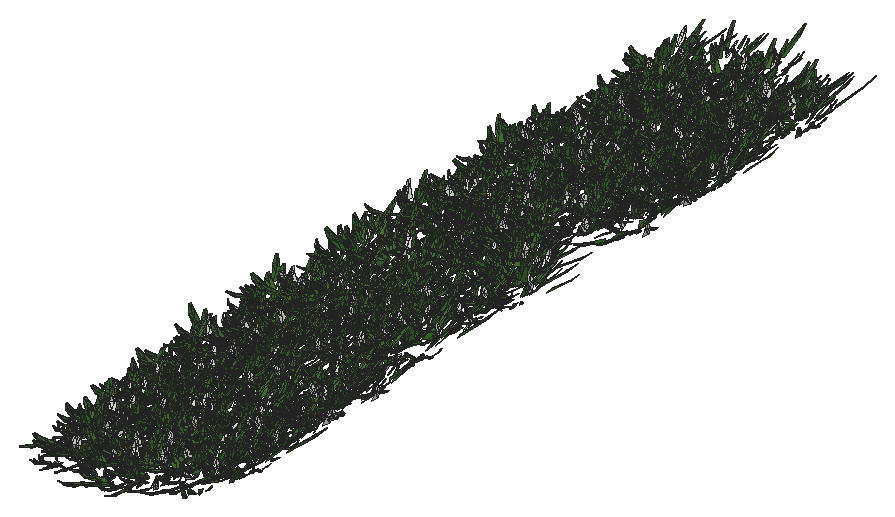
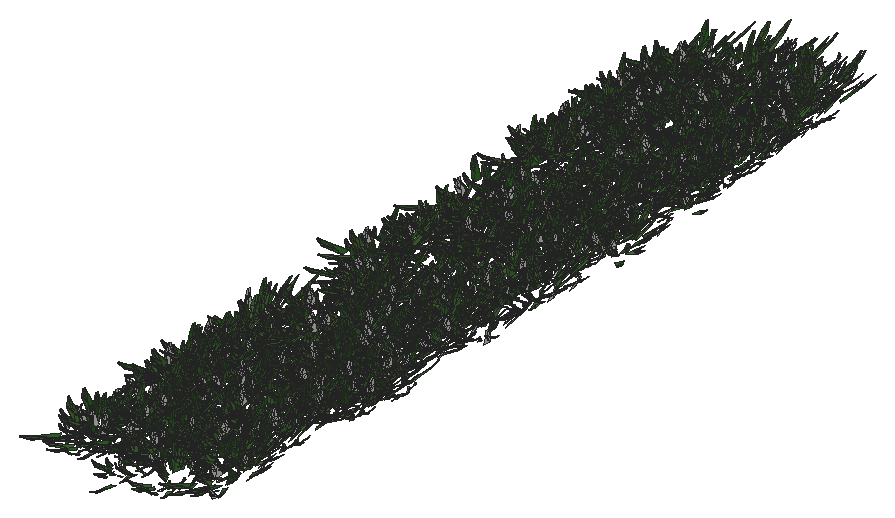
# SketchUp Ruby script. Lengths in inches.
U = 1.inch
M = Sketchup.active_model
def pt(a) = Geom::Point3d.new(a.map { |v| v * U })
def face(e, loops, mat)
  f = e.add_face(loops[0].map { |a| pt(a) })
  loops[1..].each { |l| e.add_face(l.map { |a| pt(a) }).erase! }
  f.material = f.back_material = mat if mat
  f
end
# faces: each face lists its corners as indices into pts; further lists are holes
def faces(e, pts, list, mat = nil) = list.each { |f| face(e, (f[0].is_a?(Array) ? f : [f]).map { |l| l.map { |i| pts[i] } }, mat) }
# xy, xz, yz: faces in a plane at the given z, y or x. An outline is a flat list of corners, or four numbers for a rectangle; further outlines are holes
def ring(l) = l.size == 4 ? [[l[0], l[1]], [l[2], l[1]], [l[2], l[3]], [l[0], l[3]]] : l.each_slice(2).to_a
def flat(e, list, mat, &to3) = list.each { |f| face(e, (f[0].is_a?(Array) ? f : [f]).map { |l| ring(l).map { |u, v| to3.(u, v) } }, mat) }
def xy(e, z, list, mat = nil) = flat(e, list, mat) { |x, y| [x, y, z] }
def xz(e, y, list, mat = nil) = flat(e, list, mat) { |x, z| [x, y, z] }
def yz(e, x, list, mat = nil) = flat(e, list, mat) { |y, z| [x, y, z] }
def lines(e, pts, list) = list.each { |a, b| e.add_line(pt(pts[a]), pt(pts[b])) }
# prism: a flat outline (further loops are holes) pulled along v
def prism(e, loops, v, mat = nil)
  f = face(e, loops, mat); d = Geom::Vector3d.new(v.map { |x| x * U })
  f.pushpull(f.normal.samedirection?(d) ? d.length : -d.length)
end
def box(e, o, s, mat = nil) = prism(e, [[o, [o[0] + s[0], o[1], o[2]], [o[0] + s[0], o[1] + s[1], o[2]], [o[0], o[1] + s[1], o[2]]]], [0, 0, s[2]], mat)
def at(x, y, z, deg = 0) = Geom::Transformation.translation(pt([x, y, z])) * Geom::Transformation.rotation(ORIGIN, Z_AXIS, deg.degrees)
def axes(o, x, y, z) = Geom::Transformation.new([*x, 0, *y, 0, *z, 0, *pt(o).to_a, 1])
def part(name) = M.definitions.add(name)
# library, detail: a bought-in or finely detailed component or shape, given as its bounding box
def library(name, o, s) = part(name).tap { |d| box(d.entities, o, s) }
def detail(e, o, s) = box(e.add_group.entities, o, s)
def put(e, d, t, mat = nil) = e.add_instance(d, t).tap { |i| i.material = mat if mat }
def group(e, t, mat = nil) = e.add_group.tap { |g| g.transformation = t; g.material = mat if mat }.entities
root = M.entities
M.materials.add("Material10").color = [48, 90, 38]
M.materials.add("Material11").color = [68, 110, 48]
M.materials.add("Material12").color = [48, 90, 48]
M.materials.add("Material13").color = [58, 110, 58]
M.materials.add("Material14").color = [58, 90, 38]
M.materials.add("Material15").color = [68, 100, 58]
M.materials.add("Material16").color = [48, 100, 38]
M.materials.add("Material9").color = [68, 110, 58]
c1 = part("grass00")
p = [[-0.6875,0.15,0],[-0.56,0.08,5.52],[-0.04,0.03,2.76],[0.48,-0.02,0],[0.35,-0.02,5.52],[-0.1,-0.14,5.52],
  [-0.12,0.65,8.37],[-0.42,0.65,8.37]]
faces(c1.entities,p,[[0,1,2,3],[3,2,4],[1,5,2],[5,4,2],[1,6,5],[4,5,6],[7,6,1]])
c2 = part("Group16\#1")
put(c2.entities,c1,axes([1.44,-0.61,-0.01],[0.05352,0.12609,0],[-0.10704,0.04543,0.07239],[0.06664,-0.02828,0.11628]),"Material12")
put(c2.entities,c1,axes([0.76,-0.15,-0.01],[0.04676,0.24062,0],[-0.23162,0.04501,0.06642],[0.0652,-0.01267,0.23595]),"Material9")
put(c2.entities,c1,axes([0.79,0.01,-0.01],[-0.00606,0.34651,0],[-0.34381,-0.00602,0.0432],[0.04319,0.00076,0.34386]))
put(c2.entities,c1,axes([1,0.23,-0.01],[-0.07192,0.31144,0],[-0.28722,-0.06632,0.1236],[0.12043,0.02781,0.29478]),"Material11")
put(c2.entities,c1,axes([1.66,0.77,-0.01],[-0.13828,0.29651,0],[-0.21551,-0.1005,0.22471],[0.20365,0.09498,0.23779]),"Material16")
put(c2.entities,c1,axes([0.6875,0.52,-0.01],[-0.18126,0.24051,0],[-0.22746,-0.17142,0.09788],[0.07817,0.05891,0.28481]),"Material11")
put(c2.entities,c1,axes([0.68,0.78,-0.01],[-0.215,0.18688,0],[-0.12385,-0.14248,0.21334],[0.13995,0.16101,0.18878]),"Material9")
put(c2.entities,c1,axes([0.56,1,-0.01],[-0.13756,0.07624,0],[-0.06159,-0.11112,0.0927],[0.04494,0.08108,0.12705]),"Material11")
put(c2.entities,c1,axes([0.2,0.64,-0.01],[-0.23729,0.07254,0],[-0.05711,-0.18681,0.153],[0.04473,0.14632,0.19535]),"Material16")
put(c2.entities,c1,axes([0.0625,0.72,-0.01],[-0.28874,0.02525,0],[-0.02179,-0.24916,0.14647],[0.01276,0.14591,0.25012]),"Material9")
put(c2.entities,c1,axes([-0.08,0.62,-0.01],[-0.34089,-0.04187,0],[0.03255,-0.26504,0.216],[-0.02633,0.21439,0.26703]),"Material16")
put(c2.entities,c1,axes([-0.34,0.98,-0.01],[-0.14314,-0.0493,0],[0.04397,-0.12769,0.06843],[-0.02228,0.0647,0.13505]),"Material16")
put(c2.entities,c1,axes([-0.87,1.45,-0.01],[-0.23488,-0.14114,0],[0.13761,-0.22901,0.06087],[-0.03135,0.05217,0.26717]))
put(c2.entities,c1,axes([-0.72,0.77,-0.01],[-0.14208,-0.13251,0],[0.07209,-0.0773,0.16301],[-0.11118,0.11922,0.1057]),"Material16")
put(c2.entities,c1,axes([-0.62,0.43,-0.01],[-0.14845,-0.21203,0],[0.18654,-0.13061,0.12304],[-0.10079,0.07057,0.22772]),"Material9")
put(c2.entities,c1,axes([-0.68,0.29,-0.01],[-0.13639,-0.32136,0],[0.31723,-0.13464,0.05579],[-0.05136,0.0218,0.34462]),"Material10")
put(c2.entities,c1,axes([-0.64,0.125,-0.01],[-0.0458,-0.23569,0],[0.22124,-0.043,0.08276],[-0.08124,0.01579,0.22538]),"Material13")
put(c2.entities,c1,axes([-1.6,-0.03,-0.01],[0.00576,-0.32897,0],[0.27526,0.00482,0.18018],[-0.18015,-0.00315,0.2753]),"Material11")
put(c2.entities,c1,axes([-1.36,-0.31,-0.01],[0.05718,-0.24765,0],[0.18172,0.04196,0.17267],[-0.16825,-0.03885,0.1865]),"Material16")
put(c2.entities,c1,axes([-1.54,-0.72,-0.01],[0.06537,-0.14017,0],[0.13555,0.06321,0.03939],[-0.0357,-0.01665,0.14956]))
put(c2.entities,c1,axes([-1.19,-0.9,-0.01],[0.09597,-0.12735,0],[0.11214,0.08451,0.07557],[-0.06035,-0.04548,0.14042]),"Material15")
put(c2.entities,c1,axes([-0.47,-0.54,-0.01],[0.11588,-0.10072,0],[0.0618,0.0711,0.12124],[-0.07953,-0.0915,0.0942]))
put(c2.entities,c1,axes([-0.47,-0.84,-0.01],[0.11927,-0.0661,0],[0.06603,0.11913,0.00646],[-0.00313,-0.00565,0.13621]),"Material11")
put(c2.entities,c1,axes([-0.38,-1.24,-0.01],[0.28037,-0.08571,0],[0.0618,0.20215,0.20315],[-0.05939,-0.19428,0.21139]),"Material15")
put(c2.entities,c1,axes([-0.06,-0.66,-0.01],[0.22719,-0.01987,0],[0.01247,0.14255,0.17758],[-0.01547,-0.17691,0.1431]),"Material14")
put(c2.entities,c1,axes([0.11,-0.89,-0.01],[0.14882,0.01828,0],[-0.01058,0.08611,0.12229],[0.01491,-0.12138,0.08676]),"Material12")
put(c2.entities,c1,axes([0.25,-0.72,-0.01],[0.20481,0.07053,0],[-0.06206,0.18022,0.10291],[0.03351,-0.0973,0.1906]),"Material12")
put(c2.entities,c1,axes([0.85,-1.42,-0.01],[0.16481,0.09904,0],[-0.09472,0.15762,0.05616],[0.02893,-0.04814,0.18389]),"Material11")
put(c2.entities,c1,axes([1.01,-1.09,-0.01],[0.21858,0.20385,0],[-0.17495,0.1876,0.15339],[0.10462,-0.11218,0.25652]),"Material16")
put(c2.entities,c1,axes([1.01,-0.71,-0.01],[0.08733,0.12473,0],[-0.06445,0.04512,0.13037],[0.1068,-0.07477,0.07867]),"Material12")
c3 = part("Group15\#1")
put(c3.entities,c2,at(0,0,0))
c4 = part("3darcstudiotree_grass00\#1")
put(c4.entities,c3,at(0,0,0))
put(root,c4,axes([911.62,507.39,12.99],[0.34,5.72697,0],[-2.64342,0.82003,-0.02967],[-0.12642,0.03922,1.57371]))
put(root,c4,axes([901.09,511.3,12.99],[1.82287,-4.38693,0],[2.28516,4.96154,-0.03691],[0.11809,0.2564,1.90749]))
put(root,c4,axes([899.3,512.19,12.99],[2.37795,-5.62127,0],[2.1378,4.72541,-0.03201],[0.10645,0.23529,1.88682]))
put(root,c4,axes([919.3,511.88,12.99],[2.50076,5.4884,0],[-2.31392,5.50908,-0.04664],[-0.12544,0.29866,1.77978]))
put(root,c4,axes([922.17,511.91,12.99],[-1.24752,4.90683,0],[-3.03213,-4.02809,-0.02835],[-0.08818,-0.11714,1.73088]))
put(root,c4,axes([905.31,513.99,12.99],[-2.27824,4.59704,0],[-2.30362,-5.96536,-0.01862],[-0.04923,-0.12749,1.90809]))
put(root,c4,axes([914.17,516,12.99],[-2.60594,2.85858,0],[-1.16429,-5.546,-0.02803],[-0.06327,-0.30136,1.92571]))
put(root,c4,axes([930.93,518.19,12.99],[3.35601,0.53822,0],[-0.22532,7.34135,-0.05051],[-0.0153,0.49834,1.91076]))
put(root,c4,axes([895.08,521.84,12.99],[-1.92991,-4.90294,0],[2.14831,-4.41857,-0.02928],[0.07464,-0.15352,1.35967]))
put(root,c4,axes([905.65,523.44,12.99],[-2.63848,-1.86566,0],[1.00702,-7.44154,-0.06046],[0.05687,-0.42027,1.48798]))
put(root,c4,axes([926,523.89,12.99],[-3.10548,-1.18132,0],[0.44818,-6.15625,-0.03971],[0.0257,-0.35297,1.4765]))
put(root,c4,axes([897.49,523.26,12.99],[-1.16449,5.45396,0],[-2.90449,-3.2404,-0.02753],[-0.10274,-0.11462,1.84121]))
put(root,c4,axes([914.51,526.17,12.99],[2.93419,-3.82384,0],[1.37593,5.51683,-0.05304],[0.12846,0.51506,1.86337]))
put(root,c4,axes([934.71,526.73,12.99],[2.24209,2.16707,0],[-1.0186,5.50663,-0.04149],[-0.08583,0.46398,1.90578]))
put(root,c4,axes([931.51,530.82,12.99],[-0.7426,-6.639,0],[2.915,-1.7037,-0.04783],[0.18057,-0.10554,1.6084]))
put(root,c4,axes([934.66,531.55,12.99],[2.98703,2.46119,0],[-1.07432,6.81293,-0.05978],[-0.06973,0.44222,1.49495]))
put(root,c4,axes([914.19,532.2,12.99],[3.29113,-0.43396,0],[0.16052,6.36086,-0.03809],[0.0103,0.40827,1.79573]))
put(root,c4,axes([926.06,532.53,12.99],[2.54195,2.07367,0],[-1.08806,6.96921,-0.03925],[-0.03862,0.24738,1.29995]))
put(root,c4,axes([917.6,531.75,12.99],[0.49074,6.09032,0],[-2.95531,1.24429,-0.0472],[-0.16503,0.06948,1.46547]))
put(root,c4,axes([897.78,535.97,12.99],[1.52125,-4.69601,0],[2.1276,3.60136,-0.04843],[0.18496,0.31307,1.72564]))
put(root,c4,axes([903.64,536.54,12.99],[2.39249,-2.44782,0],[1.16829,5.96659,-0.04939],[0.0929,0.47446,1.80606]))
put(root,c4,axes([895.21,535.38,12.99],[-0.41215,7.13038,0],[-3.37299,-1.01874,-0.03274],[-0.10036,-0.03031,1.44297]))
put(root,c4,axes([911.05,535.47,12.99],[-1.79373,6.75105,0],[-2.77607,-3.8541,-0.06137],[-0.17197,-0.23875,1.46064]))
put(root,c4,axes([923.03,540.81,12.99],[2.70825,1.08108,0],[-0.55903,7.3176,-0.04039],[-0.02179,0.2852,1.39779]))
put(root,c4,axes([926.1,541.03,12.99],[3.0266,-0.27277,0],[0.11405,6.61218,-0.03451],[0.00641,0.37148,1.8714]))
put(root,c4,axes([896.8,540.54,12.99],[0.57317,6.39839,0],[-3.07282,1.43831,-0.02758],[-0.10194,0.04772,1.62317]))
put(root,c4,axes([894.13,542.98,12.99],[-0.04355,-5.68696,0],[3.06634,-0.12269,-0.04239],[0.1434,-0.00574,1.42343]))
put(root,c4,axes([935.43,543.85,12.99],[1.14678,-5.5994,0],[2.21293,2.36815,-0.04141],[0.22096,0.23646,1.97468]))
put(root,c4,axes([910.25,543.03,12.99],[-0.07356,6.6061,0],[-2.87925,-0.16752,-0.03168],[-0.13306,-0.00774,1.66016]))
put(root,c4,axes([916.99,545.44,12.99],[-0.22644,-5.7932,0],[3.1204,-0.63732,-0.01785],[0.07882,-0.0161,1.90542]))
put(root,c4,axes([901.99,546.02,12.99],[-2.22727,-5.99191,0],[2.4648,-4.78734,-0.06095],[0.18437,-0.35809,1.76096]))
put(root,c4,axes([908.8,549.42,12.99],[-1.36063,-6.84812,0],[2.89693,-3.00754,-0.02239],[0.08865,-0.09204,1.89813]))
put(root,c4,axes([922.76,551.22,12.99],[2.82961,-3.8496,0],[1.56723,6.01934,-0.02674],[0.04894,0.18795,1.50406]))
put(root,c4,axes([925.56,552.73,12.99],[2.24091,-5.60604,0],[1.99594,4.16889,-0.04297],[0.12661,0.26444,1.48019]))
put(root,c4,axes([893.13,553.17,12.99],[1.46268,-6.84801,0],[2.66295,2.97202,-0.03421],[0.14319,0.15981,1.89316]))
put(root,c4,axes([933.37,554.94,12.99],[-1.60421,-6.26587,0],[2.10282,-2.81311,-0.0221],[0.10402,-0.13915,1.82262]))
put(root,c4,axes([899.48,555.6,12.99],[-0.27492,-6.2516,0],[2.80374,-0.64426,-0.02999],[0.1475,-0.03389,1.91089]))
put(root,c4,axes([901.93,554.68,12.99],[-2.10162,2.80691,0],[-1.6179,-6.32971,-0.05376],[-0.08517,-0.33321,1.38154]))
put(root,c4,axes([931.97,558.13,12.99],[1.20273,-5.08222,0],[2.87348,3.55326,-0.03985],[0.11745,0.14524,1.5017]))
put(root,c4,axes([910.82,559.6,12.99],[2.65553,-1.98837,0],[0.86174,6.01359,-0.03684],[0.04886,0.34099,1.61813]))
put(root,c4,axes([919.3,559.79,12.99],[-0.92876,-5.81291,0],[2.33925,-1.95294,-0.03784],[0.17266,-0.14414,1.65933]))
put(root,c4,axes([899.22,560.83,12.99],[0.14872,-5.87734,0],[2.84203,0.37577,-0.03098],[0.1244,0.01645,1.57088]))
put(root,c4,axes([893.03,560.92,12.99],[-0.76721,-6.56598,0],[2.80308,-1.71142,-0.04991],[0.16056,-0.09803,1.32514]))
put(root,c4,axes([901.87,563.86,12.99],[0.86779,-6.44688,0],[3.29606,2.31828,-0.02541],[0.07611,0.05354,1.48254]))
put(root,c4,axes([925.49,564.01,12.99],[3.00912,-1.86696,0],[0.83394,7.02336,-0.0215],[0.02203,0.18551,1.70776]))
put(root,c4,axes([933.42,564.83,12.99],[-2.81152,-3.41489,0],[1.39335,-5.99415,-0.03648],[0.07534,-0.32411,1.79293]))
put(root,c4,axes([913.24,567.95,12.99],[2.91119,-3.41984,0],[1.58451,7.04797,-0.04443],[0.05964,0.26528,1.39643]))
put(root,c4,axes([930.81,568.44,12.99],[1.07755,-6.0652,0],[2.75492,2.55744,-0.04502],[0.19028,0.17664,1.86083]))
put(root,c4,axes([898.57,570.125,12.99],[0.66031,-7.75823,0],[2.98052,1.3255,-0.02432],[0.08896,0.03956,1.55217]))
put(root,c4,axes([903.51,568.01,12.99],[-2.55136,-0.37019,0],[0.21266,-7.65835,-0.04372],[0.00789,-0.28423,1.31241]))
put(root,c4,axes([892.51,568.625,12.99],[-2.70337,4.4882,0],[-1.55371,-4.89002,-0.02785],[-0.08332,-0.26224,1.84622]))
put(root,c4,axes([906.42,572.39,12.99],[0.82047,6.51109,0],[-2.65358,1.74721,-0.02733],[-0.11397,0.07504,1.64375]))
put(root,c4,axes([934.53,573.93,12.99],[-1.61582,-5.04917,0],[2.30469,-3.85382,-0.02018],[0.07529,-0.12589,1.81061]))
put(root,c4,axes([909.06,573.86,12.99],[1.03892,6.48849,0],[-2.96707,2.4824,-0.03042],[-0.10595,0.08864,1.60735]))
put(root,c4,axes([917.76,577.75,12.99],[2.83159,1.20572,0],[-0.46618,5.72066,-0.03922],[-0.03004,0.36868,1.46066]))
put(root,c4,axes([927.84,578.64,12.99],[-0.05016,-6.74869,0],[3.47924,-0.13511,-0.0635],[0.25664,-0.00997,1.92948]))
put(root,c4,axes([903.48,577.58,12.99],[-2.8288,-1.01098,0],[0.5257,-7.68597,-0.04342],[0.02399,-0.35073,1.66984]))
put(root,c4,axes([907.71,577.89,12.99],[0.7383,7.4918,0],[-2.86561,1.4756,-0.04632],[-0.17959,0.09248,1.6013]))
put(root,c4,axes([898.29,578.13,12.99],[-3.47147,0.94023,0],[-0.34005,-6.56028,-0.03012],[-0.01166,-0.22504,1.30483]))
put(root,c4,axes([913.85,580.83,12.99],[2.85458,-2.4144,0],[0.90082,5.56514,-0.04569],[0.07926,0.48966,1.78027]))
put(root,c4,axes([895.07,582.8,12.99],[-0.07151,5.57846,0],[-2.5198,-0.16879,-0.04664],[-0.191,-0.01279,1.41669]))
put(root,c4,axes([902.39,589.33,12.99],[-2.87948,-2.17383,0],[0.90398,-6.25682,-0.04962],[0.07103,-0.49164,1.8049]))
put(root,c4,axes([919.75,591.55,12.99],[2.81213,-4.07835,0],[1.6403,5.90987,-0.04672],[0.11008,0.39661,1.84728]))
put(root,c4,axes([913.87,591,12.99],[-1.55553,-5.63634,0],[2.69451,-3.88567,-0.04882],[0.13072,-0.18851,1.38366]))
put(root,c4,axes([926.78,593.01,12.99],[0.94413,-7.19204,0],[2.66579,1.82856,-0.0465],[0.16992,0.11655,1.45674]))
put(root,c4,axes([923.21,591.68,12.99],[2.50014,4.15141,0],[-1.81588,5.71425,-0.05492],[-0.12483,0.39281,1.63919]))
put(root,c4,axes([890.46,595.94,12.99],[-1.39258,5.37899,0],[-2.78969,-3.77383,-0.04665],[-0.1335,-0.18059,1.47851]))
put(root,c4,axes([931.64,597.86,12.99],[3.08666,3.01957,0],[-1.37734,7.35682,-0.06274],[-0.09879,0.52768,1.92197]))
put(root,c4,axes([922.87,601.0625,12.99],[3.40345,0.80319,0],[-0.35208,7.79564,-0.06196],[-0.02083,0.46114,1.53928]))
put(root,c4,axes([896.75,599.38,12.99],[-2.37919,1.70232,0],[-0.98908,-7.22313,-0.0251],[-0.02634,-0.19235,1.59541]))
put(root,c4,axes([910.33,600.22,12.99],[1.27071,7.43264,0],[-2.73445,2.44274,-0.05423],[-0.17184,0.15351,1.37014]))
put(root,c4,axes([914.18,601.01,12.99],[-2.71794,-2.84239,0],[1.0724,-5.35819,-0.02741],[0.0602,-0.30081,1.86713]))
put(root,c4,axes([907.29,602.4375,12.99],[3.09734,3.11798,0],[-1.07985,5.60512,-0.04159],[-0.06485,0.33661,1.42181]))
put(root,c4,axes([901.5625,600.88,12.99],[-0.67912,7.33073,0],[-3.23912,-1.56795,-0.05285],[-0.196,-0.09488,1.72177]))
put(root,c4,axes([895.03,602.25,12.99],[2.06342,5.41056,0],[-1.85953,3.70556,-0.0286],[-0.1154,0.22996,1.81122]))
put(root,c4,axes([921.49,605.92,12.99],[1.54134,-4.78126,0],[2.32684,3.91946,-0.04551],[0.15187,0.25581,1.64335]))
put(root,c4,axes([914.17,605.18,12.99],[-1.50632,-4.69201,0],[2.73865,-4.59409,-0.05528],[0.17049,-0.28599,1.78248]))
put(root,c4,axes([919.71,607.39,12.99],[-3.46773,-1.02932,0],[0.4256,-7.49196,-0.02421],[0.01142,-0.20095,1.66024]))
put(root,c4,axes([910.52,608.8,12.99],[-2.49845,-5.44109,0],[2.40238,-5.76411,-0.03405],[0.07195,-0.17263,1.46358]))
put(root,c4,axes([894.73,610.01,12.99],[-0.0959,-6.54768,0],[3.1318,-0.23968,-0.02714],[0.09123,-0.00698,1.44559]))
put(root,c4,axes([901.81,609.875,12.99],[-2.1387,-4.22142,0],[1.73135,-4.58332,-0.01919],[0.06882,-0.18218,1.99409]))
put(root,c4,axes([929.98,611.28,12.99],[-0.93481,-5.37778,0],[2.82075,-2.56208,-0.04918],[0.14755,-0.13402,1.34418]))
put(root,c4,axes([917.01,616.94,12.99],[2.59771,-2.31669,0],[0.88695,5.19669,-0.03886],[0.06413,0.37576,1.52001]))
put(root,c4,axes([923.46,615.26,12.99],[-2.73622,0.78622,0],[-0.41112,-7.47622,-0.04842],[-0.02602,-0.47315,1.94818]))
put(root,c4,axes([930.31,619.48,12.99],[0.40616,-5.59706,0],[3.26818,1.23923,-0.06063],[0.20259,0.07682,1.53907]))
put(root,c4,axes([899.28,625.21,12.99],[1.48607,-6.00699,0],[2.71444,3.50888,-0.04614],[0.13946,0.18028,1.48544]))
put(root,c4,axes([928.17,625.99,12.99],[2.65845,-2.85345,0],[1.05816,5.15125,-0.03796],[0.07227,0.35184,1.52986]))
put(root,c4,axes([891.27,623.87,12.99],[0.1348,6.56883,0],[-3.04635,0.32665,-0.04808],[-0.19581,0.021,1.70557]))
put(root,c4,axes([911.5625,625.78,12.99],[1.96904,6.36442,0],[-2.63699,4.26294,-0.03132],[-0.10336,0.16709,1.7905]))
put(root,c4,axes([902.68,625.72,12.99],[-1.44847,7.20412,0],[-2.84419,-2.98807,-0.02861],[-0.11414,-0.11991,1.88512]))
put(root,c4,axes([917.68,628.26,12.99],[1.92859,6.40127,0],[-2.1329,3.35776,-0.04649],[-0.14033,0.22092,1.30192]))
put(root,c4,axes([892.55,628.5,12.99],[0.7965,6.40774,0],[-3.08556,2.00411,-0.01918],[-0.07901,0.05132,1.88463]))
put(root,c4,axes([933.56,634.16,12.99],[3.0297,-0.61474,0],[0.27475,7.07526,-0.01913],[0.00739,0.1902,1.86132]))
put(root,c4,axes([909.38,635.46,12.99],[2.96081,2.71039,0],[-1.11902,6.38738,-0.05201],[-0.08237,0.47016,1.75905]))
put(root,c4,axes([899.58,638.61,12.99],[-2.68453,-4.05111,0],[1.51474,-5.2449,-0.0411],[0.0862,-0.29848,1.43569]))
put(root,c4,axes([927.57,637.76,12.99],[-0.5928,7.42861,0],[-3.44276,-1.43553,-0.02378],[-0.09545,-0.0398,1.95907]))
put(root,c4,axes([899.32,642.41,12.99],[2.59926,-1.54725,0],[0.69692,6.11752,-0.03218],[0.02822,0.24776,1.32043]))
put(root,c4,axes([927.82,642.72,12.99],[3.30378,0.12998,0],[-0.05244,6.96435,-0.04862],[-0.00279,0.3699,1.39123]))
put(root,c4,axes([911.83,642.75,12.99],[-1.81939,4.62689,0],[-2.16643,-4.4513,-0.05045],[-0.13948,-0.28658,1.48531]))
put(root,c4,axes([918.25,646.97,12.99],[1.07125,-5.88046,0],[2.56502,2.44161,-0.04485],[0.17282,0.1645,1.59096]))
put(root,c4,axes([923.6875,649.01,12.99],[2.65984,-5.15497,0],[1.88895,5.09277,-0.04452],[0.14052,0.37886,1.95574]))
put(root,c4,axes([913.17,646.6875,12.99],[0.28785,6.1866,0],[-3.00356,0.73023,-0.05804],[-0.19462,0.04732,1.39706]))
put(root,c4,axes([903.36,648.48,12.99],[-0.63085,-5.64288,0],[2.60325,-1.52071,-0.03508],[0.17624,-0.10295,1.91126]))
put(root,c4,axes([890.6,648.84,12.99],[1.84408,4.39499,0],[-2.00782,4.40201,-0.02632],[-0.0972,0.2131,1.95302]))
put(root,c4,axes([917.4375,652.04,12.99],[-2.91275,-0.75216,0],[0.38619,-7.81446,-0.03054],[0.01335,-0.27005,1.83699]))
put(root,c4,axes([911.56,652.36,12.99],[-1.13216,5.99058,0],[-2.90662,-2.87034,-0.05011],[-0.17897,-0.17673,1.6899]))
put(root,c4,axes([896.78,652.61,12.99],[-2.03571,3.61595,0],[-2.1162,-6.22521,-0.03993],[-0.10032,-0.29512,1.9372]))
put(root,c4,axes([922.5,653.11,12.99],[-1.29988,5.1822,0],[-2.7348,-3.58444,-0.01882],[-0.07351,-0.09635,1.94745]))
put(root,c4,axes([895.15,656.34,12.99],[-0.51283,6.72965,0],[-2.43312,-0.96883,-0.03897],[-0.20137,-0.08018,1.77692]))
put(root,c4,axes([903.2,657.31,12.99],[-1.40266,4.89142,0],[-2.06635,-3.09618,-0.04],[-0.144,-0.21577,1.45882]))
put(root,c4,axes([902.09,662.7,12.99],[3.16941,3.18482,0],[-1.18871,6.18123,-0.02572],[-0.03758,0.1954,1.47108]))
put(root,c4,axes([913.77,662.91,12.99],[-2.68051,-1.51269,0],[0.75808,-7.01918,-0.03453],[0.02765,-0.25599,1.44935]))
put(root,c4,axes([906.33,664.2,12.99],[3.0336,3.04139,0],[-1.16472,6.07032,-0.04488],[-0.08957,0.46682,1.97665]))
put(root,c4,axes([926.74,666.3125,12.99],[2.11569,-2.99429,0],[1.59473,5.88776,-0.03178],[0.06665,0.24606,1.65559]))
put(root,c4,axes([908.91,666.86,12.99],[2.25666,-3.63006,0],[1.90685,6.19401,-0.04926],[0.1204,0.3911,1.93034]))
put(root,c4,axes([896.61,664.625,12.99],[-3.12012,1.25449,0],[-0.45282,-5.88484,-0.03096],[-0.02076,-0.26978,1.38775]))
put(root,c4,axes([919.59,665.59,12.99],[-1.67076,5.85031,0],[-2.79261,-4.16727,-0.02867],[-0.09365,-0.13975,1.78429]))
put(root,c4,axes([902.98,672.4,12.99],[2.72155,-0.38084,0],[0.21032,7.85341,-0.0507],[0.01092,0.40767,1.66388]))
put(root,c4,axes([894.3,671.6,12.99],[-0.62276,6.69378,0],[-3.04855,-1.48199,-0.02719],[-0.11164,-0.05427,1.79436]))
put(root,c4,axes([925.32,672.68,12.99],[1.07616,6.01364,0],[-3.17679,2.97053,-0.06498],[-0.24678,0.23076,1.93183]))
put(root,c4,axes([919.6875,676.73,12.99],[1.94818,-4.88856,0],[2.58666,5.38633,-0.04921],[0.12638,0.26317,1.66765]))
put(root,c4,axes([934.8125,675.58,12.99],[-1.57713,-4.59348,0],[2.5508,-4.57622,-0.04646],[0.14939,-0.26801,1.81816]))
put(root,c4,axes([909.14,674.83,12.99],[-3.15765,-1.46964,0],[0.65595,-7.36428,-0.03896],[0.03047,-0.34213,1.76791]))
put(root,c4,axes([890.86,681.53,12.99],[3.02413,-2.56039,0],[0.88869,5.48468,-0.03178],[0.05674,0.35016,1.80429]))
put(root,c4,axes([931.99,682.82,12.99],[0.33709,-7.51808,0],[3.33483,0.78129,-0.06373],[0.20711,0.04852,1.50237]))
put(root,c4,axes([909.91,682.99,12.99],[3.11749,-1.17569,0],[0.43678,6.05167,-0.03976],[0.03098,0.4293,1.7619]))
put(root,c4,axes([905.9375,685.55,12.99],[3.04853,0.43387,0],[-0.17111,6.28235,-0.04181],[-0.01342,0.49279,1.95138]))
put(root,c4,axes([903.07,684.24,12.99],[-3.06718,1.52954,0],[-0.63631,-6.66731,-0.03649],[-0.03425,-0.35892,1.80375]))
put(root,c4,axes([893.66,684.98,12.99],[-2.36593,3.79228,0],[-1.55094,-5.05591,-0.04222],[-0.115,-0.3749,1.75818]))
put(root,c4,axes([912.96,686.46,12.99],[0.61013,6.83732,0],[-2.52423,1.17698,-0.03877],[-0.20843,0.09719,1.93915]))
put(root,c4,axes([922.17,689.91,12.99],[3.22326,0.89472,0],[-0.31531,5.93539,-0.01966],[-0.0118,0.2222,1.78732]))
put(root,c4,axes([917.72,689.15,12.99],[0.32638,6.89253,0],[-3.39947,0.84112,-0.03135],[-0.10183,0.02519,1.53244]))
put(root,c4,axes([926.53,690.14,12.99],[1.5341,4.31893,0],[-2.19599,4.07581,-0.04172],[-0.14897,0.2765,1.78477]))
put(root,c4,axes([931.74,691.2,12.99],[-1.65035,-5.60764,0],[2.65125,-4.07709,-0.0439],[0.12847,-0.19756,1.54604]))
put(root,c4,axes([909.13,690.54,12.99],[-2.16713,3.63075,0],[-1.95024,-6.08247,-0.02359],[-0.05145,-0.16047,1.66971]))
put(root,c4,axes([892.85,693.65,12.99],[-0.68411,-6.20035,0],[2.75809,-1.59009,-0.02503],[0.09196,-0.05302,1.47852]))
put(root,c4,axes([898.97,694.76,12.99],[3.02577,0.05138,0],[-0.02136,6.57245,-0.04293],[-0.0011,0.33717,1.35522]))
put(root,c4,axes([934.35,694.45,12.99],[-2.4329,-3.38946,0],[1.33089,-4.9916,-0.03312],[0.08401,-0.3151,1.70984]))
put(root,c4,axes([891.26,695.03,12.99],[-2.37214,-2.81798,0],[1.12361,-4.94224,-0.02241],[0.05211,-0.22923,1.68548]))
put(root,c4,axes([925.62,700.17,12.99],[2.55004,0.56137,0],[-0.26222,6.22398,-0.03978],[-0.02007,0.47634,1.9745]))
put(root,c4,axes([931.01,699.98,12.99],[-1.50806,-4.47998,0],[2.32582,-4.09096,-0.03027],[0.08802,-0.15482,1.47708]))
put(root,c4,axes([913.54,699.125,12.99],[-3.04603,-1.16193,0],[0.4841,-6.63127,-0.03361],[0.02113,-0.28941,1.54092]))
put(root,c4,axes([907.11,702.15,12.99],[1.77944,4.32296,0],[-1.81202,3.89734,-0.04643],[-0.17338,0.37292,1.7498]))
put(root,c4,axes([923.24,702.73,12.99],[-3.03678,-2.70559,0],[1.03947,-6.09632,-0.03755],[0.05411,-0.31736,1.55797]))
put(root,c4,axes([934.91,704.35,12.99],[2.64478,0.95853,0],[-0.48752,7.02874,-0.02805],[-0.02052,0.29581,1.99488]))
put(root,c4,axes([898.26,703.16,12.99],[-3.0366,-0.20239,0],[0.07296,-5.72024,-0.0193],[0.00327,-0.25623,1.99558]))
put(root,c4,axes([927.08,707.95,12.99],[0.69865,-7.14504,0],[3.01104,1.53843,-0.0396],[0.13562,0.06929,1.48525]))
put(root,c4,axes([934.12,709.98,12.99],[0.73418,-6.79452,0],[2.93095,1.65485,-0.04714],[0.14849,0.08384,1.34372]))
put(root,c4,axes([923.46,710.54,12.99],[-0.33358,-5.71393,0],[3.12378,-0.95292,-0.03174],[0.12939,-0.03947,1.77768]))
put(root,c4,axes([910.09,711.41,12.99],[2.38498,-2.21708,0],[0.97992,5.50805,-0.02601],[0.04038,0.22696,1.4702]))
put(root,c4,axes([913.18,710.68,12.99],[-2.10641,-2.92137,0],[1.6011,-6.03227,-0.04577],[0.10991,-0.4141,1.96036]))
put(root,c4,axes([919.04,712.79,12.99],[1.76737,-4.42523,0],[2.23598,4.66622,-0.05494],[0.17934,0.37427,1.83588]))
put(root,c4,axes([901.86,711.63,12.99],[-2.70739,2.98432,0],[-1.16274,-5.51181,-0.02015],[-0.04497,-0.21316,1.88684]))
put(root,c4,axes([899.58,713.57,12.99],[-0.0319,6.7723,0],[-3.49626,-0.08606,-0.05791],[-0.19427,-0.00478,1.60897]))
put(root,c4,axes([919.59,718.64,12.99],[-0.20897,-7.41009,0],[3.42426,-0.50459,-0.03565],[0.1157,-0.01705,1.53082]))
put(root,c4,axes([895.26,718.29,12.99],[-2.71333,-4.1599,0],[1.39332,-4.74872,-0.03319],[0.08815,-0.30045,1.63594]))
put(root,c4,axes([930.71,718.5,12.99],[2.52749,4.89001,0],[-1.97629,5.33749,-0.04954],[-0.13616,0.36773,1.78537]))
put(root,c4,axes([923.56,721.11,12.99],[-1.83593,-6.76701,0],[2.50173,-3.54653,-0.05324],[0.20696,-0.29339,1.84703]))
put(root,c4,axes([905.46,721.41,12.99],[1.80116,6.23947,0],[-2.08606,3.14656,-0.04277],[-0.16521,0.24919,1.58679]))
put(root,c4,axes([925.51,721.92,12.99],[-1.8938,3.66251,0],[-2.15423,-5.8204,-0.04396],[-0.11313,-0.30567,1.82298]))
put(root,c4,axes([902.79,722.73,12.99],[-0.06993,7.72932,0],[-3.42655,-0.16199,-0.04199],[-0.1504,-0.00711,1.68448]))
put(root,c4,axes([901.97,727.43,12.99],[3.06249,-2.4311,0],[1.08782,7.16037,-0.03586],[0.04665,0.30704,1.80381]))
put(root,c4,axes([907.18,727.99,12.99],[1.63097,-4.20307,0],[2.47724,5.02288,-0.037],[0.09316,0.1889,1.52862]))
put(root,c4,axes([925.5625,726.54,12.99],[-2.27086,5.66663,0],[-2.2045,-4.61617,-0.02313],[-0.08047,-0.1685,1.93523]))
put(root,c4,axes([897.14,729.58,12.99],[-2.25828,-3.34609,0],[1.52601,-5.38148,-0.04254],[0.1076,-0.37945,1.78955]))
put(root,c4,axes([914.8,729.87,12.99],[-3.32554,0.64782,0],[-0.23181,-6.21804,-0.04489],[-0.01897,-0.50881,1.86365]))
put(root,c4,axes([921.75,732.87,12.99],[2.57149,2.9871,0],[-1.53335,6.89734,-0.02666],[-0.0386,0.17364,1.48409]))
put(root,c4,axes([894.45,731.125,12.99],[-2.03428,3.10598,0],[-1.53915,-5.26739,-0.04884],[-0.09906,-0.339,1.38796]))
put(root,c4,axes([933.46,736.09,12.99],[2.60169,4.35909,0],[-1.89558,5.9116,-0.04132],[-0.10454,0.32602,1.88254]))
put(root,c4,axes([913.16,737.38,12.99],[2.54546,1.14859,0],[-0.52438,6.07227,-0.02055],[-0.02011,0.23285,1.87683]))
put(root,c4,axes([910.98,738.49,12.99],[3.14751,-2.04846,0],[0.80017,6.42436,-0.0361],[0.03698,0.29692,1.4995]))
put(root,c4,axes([893.2,738.78,12.99],[2.64912,1.70625,0],[-0.90902,7.37458,-0.04858],[-0.0451,0.36588,1.57379]))
put(root,c4,axes([924.09,736.66,12.99],[-2.60145,4.40679,0],[-1.83185,-5.65051,-0.03727],[-0.09886,-0.30493,1.88005]))
put(root,c4,axes([927.4,740.69,12.99],[-2.00765,-5.98954,0],[2.59722,-4.54893,-0.04805],[0.13739,-0.24064,1.61679]))
put(root,c4,axes([931.9,740.5625,12.99],[-3.15604,0.22694,0],[-0.08455,-6.1438,-0.03177],[-0.00537,-0.39057,1.98473]))
put(root,c4,axes([902.65,746.13,12.99],[-1.17967,-4.89582,0],[3.04698,-3.83627,-0.06742],[0.19561,-0.24628,1.58058]))
put(root,c4,axes([913.52,747.39,12.99],[0.18692,6.5512,0],[-2.68,0.39955,-0.03468],[-0.16182,0.02412,1.72254]))
